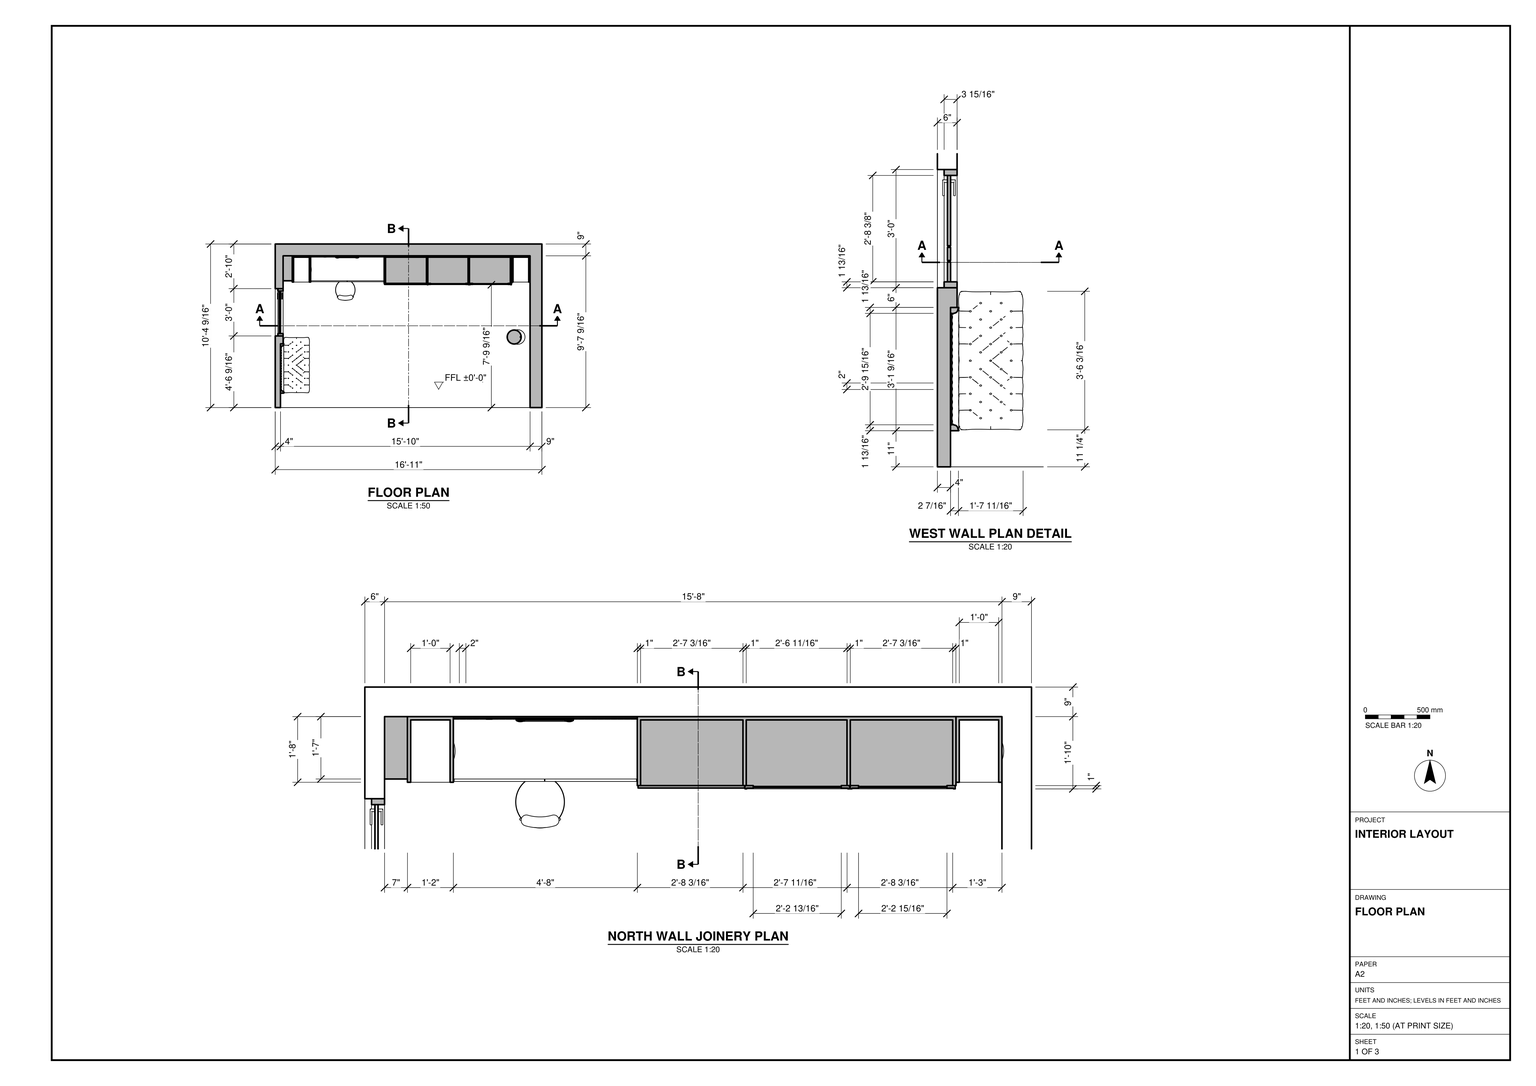
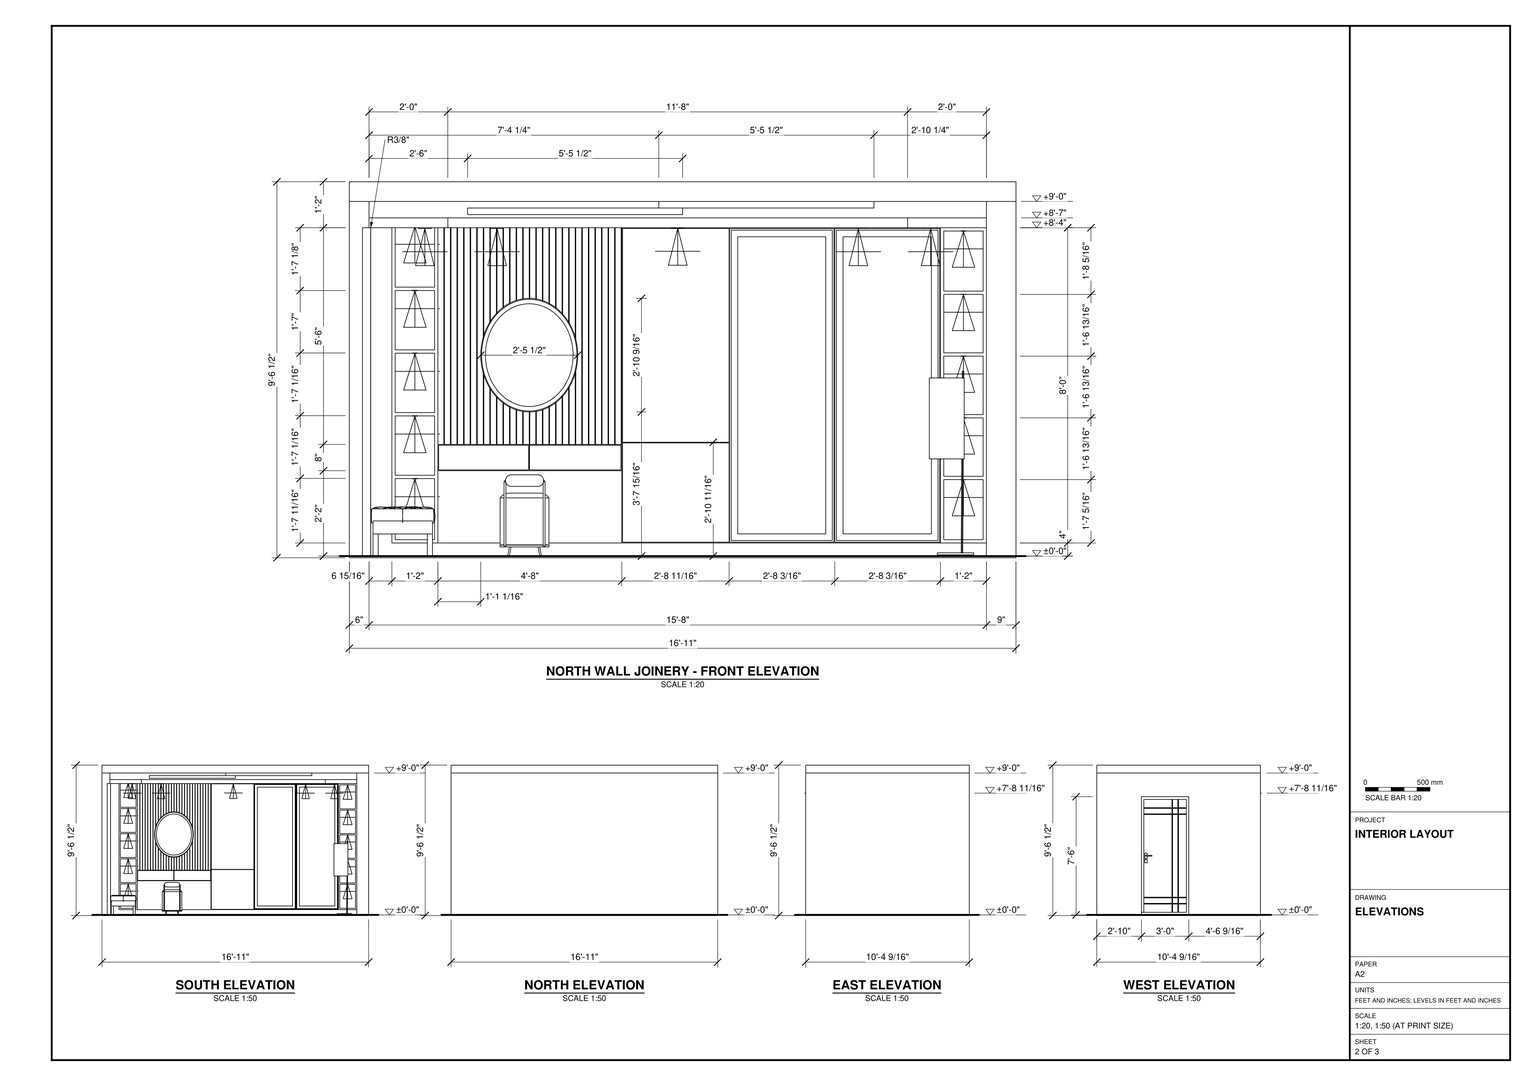
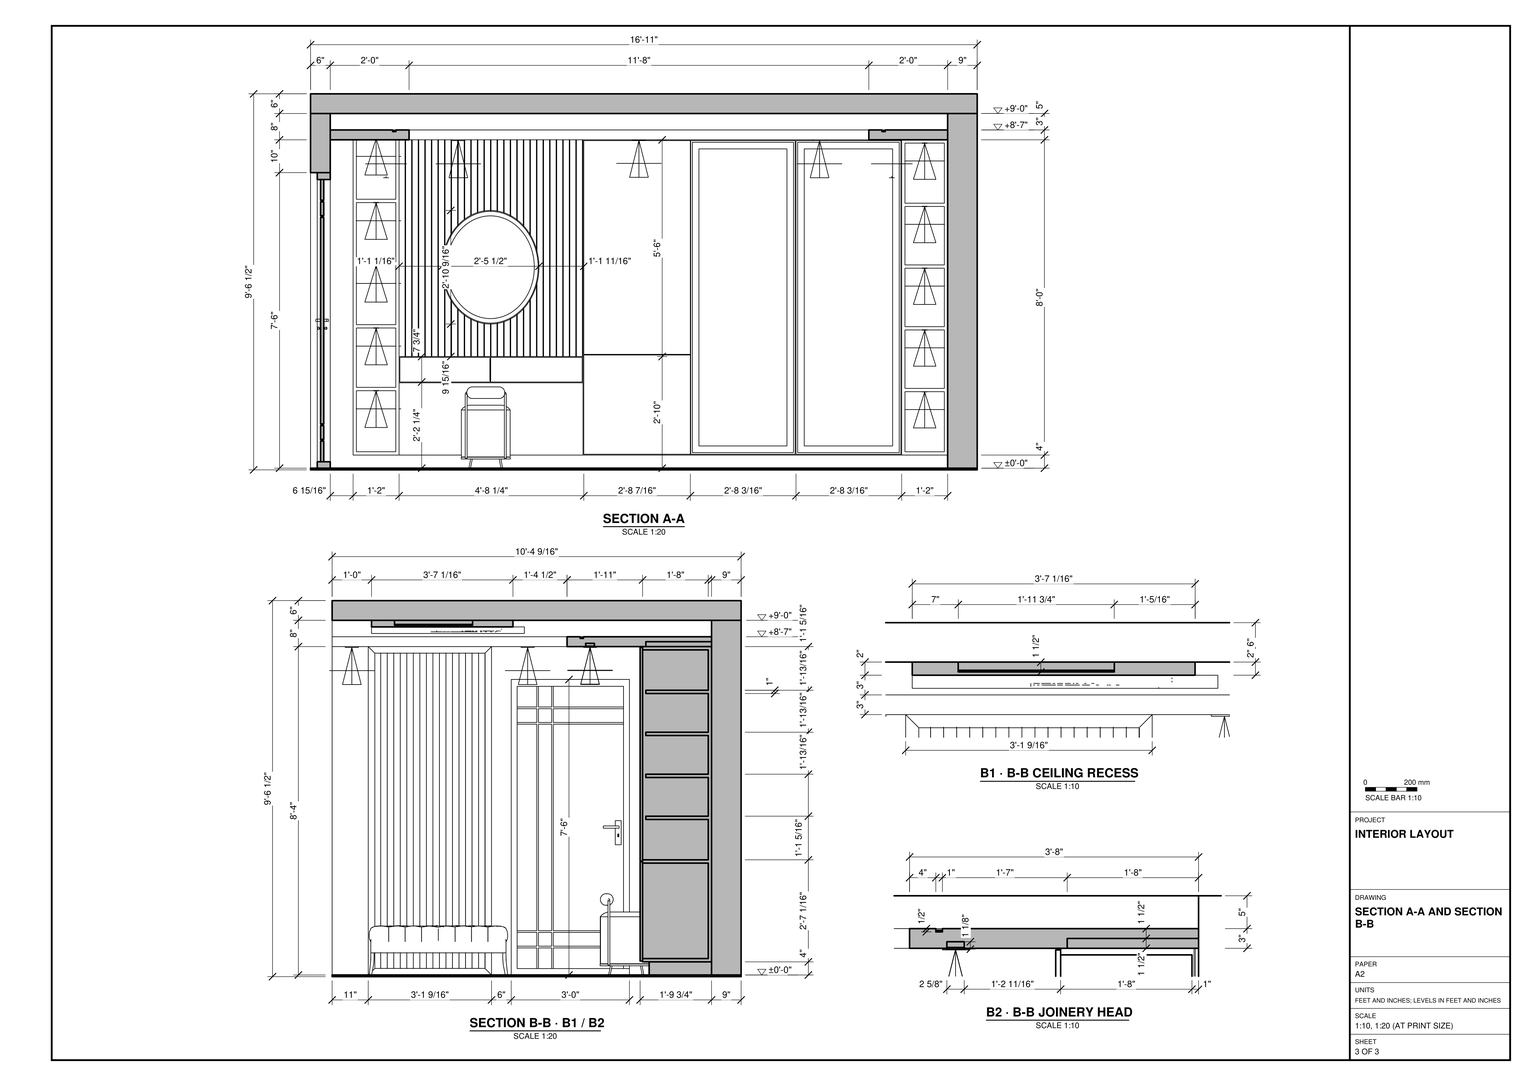
Work in feet and inches in SketchUp. Use task_files/diagram_01.pdf to model the dressing room. Set the finished floor at ±0'-0". The overall size is 16'-11" east to west, 10'-4 9/16" north to south and 9'-6 1/2" high.

Build the floor, the north, east and west walls, and the ceiling slab. Follow the wall thicknesses in plan and leave the south side open as drawn. Fit the door in the west wall, with the bench and its vertical slatted backing on the south side of the door.

Use the north wall joinery plan for cabinet depths and the front elevation for the arrangement of the bays. Model the dressing counter with drawers, knee space, a seat and a mirror on slatted backing. Continue the run with the tall cupboards and include the narrow open shelving at both ends. Use the sections to shape the plinth, joinery head and stepped ceiling recess. Place the lights as shown. Decor and loose items may be any suitable library components.

Keep shell elements and individual furniture and joinery pieces in separate groups or components, and use components for repeated parts. Save one SketchUp model as output_files/dressing_room_with_fitted_wardrobes_and_a_vanity.skp.

# SketchUp Ruby script. Lengths in inches.
U = 1.inch
M = Sketchup.active_model
def pt(a) = Geom::Point3d.new(a.map { |v| v * U })
def face(e, loops, mat)
  f = e.add_face(loops[0].map { |a| pt(a) })
  loops[1..].each { |l| e.add_face(l.map { |a| pt(a) }).erase! }
  f.material = f.back_material = mat if mat
  f
end
# faces: each face lists its corners as indices into pts; further lists are holes
def faces(e, pts, list, mat = nil) = list.each { |f| face(e, (f[0].is_a?(Array) ? f : [f]).map { |l| l.map { |i| pts[i] } }, mat) }
# xy, xz, yz: faces in a plane at the given z, y or x. An outline is a flat list of corners, or four numbers for a rectangle; further outlines are holes
def ring(l) = l.size == 4 ? [[l[0], l[1]], [l[2], l[1]], [l[2], l[3]], [l[0], l[3]]] : l.each_slice(2).to_a
def flat(e, list, mat, &to3) = list.each { |f| face(e, (f[0].is_a?(Array) ? f : [f]).map { |l| ring(l).map { |u, v| to3.(u, v) } }, mat) }
def xy(e, z, list, mat = nil) = flat(e, list, mat) { |x, y| [x, y, z] }
def xz(e, y, list, mat = nil) = flat(e, list, mat) { |x, z| [x, y, z] }
def yz(e, x, list, mat = nil) = flat(e, list, mat) { |y, z| [x, y, z] }
def lines(e, pts, list) = list.each { |a, b| e.add_line(pt(pts[a]), pt(pts[b])) }
# prism: a flat outline (further loops are holes) pulled along v
def prism(e, loops, v, mat = nil)
  f = face(e, loops, mat); d = Geom::Vector3d.new(v.map { |x| x * U })
  f.pushpull(f.normal.samedirection?(d) ? d.length : -d.length)
end
def box(e, o, s, mat = nil) = prism(e, [[o, [o[0] + s[0], o[1], o[2]], [o[0] + s[0], o[1] + s[1], o[2]], [o[0], o[1] + s[1], o[2]]]], [0, 0, s[2]], mat)
def at(x, y, z, deg = 0) = Geom::Transformation.translation(pt([x, y, z])) * Geom::Transformation.rotation(ORIGIN, Z_AXIS, deg.degrees)
def axes(o, x, y, z) = Geom::Transformation.new([*x, 0, *y, 0, *z, 0, *pt(o).to_a, 1])
def part(name) = M.definitions.add(name)
# library, detail: a bought-in or finely detailed component or shape, given as its bounding box
def library(name, o, s) = part(name).tap { |d| box(d.entities, o, s) }
def detail(e, o, s) = box(e.add_group.entities, o, s)
def put(e, d, t, mat = nil) = e.add_instance(d, t).tap { |i| i.material = mat if mat }
def group(e, t, mat = nil) = e.add_group.tap { |g| g.transformation = t; g.material = mat if mat }.entities
root = M.entities
M.materials.add("0001 AP 9436 AIR BREEZE").color = [243, 237, 232]
M.materials.add("[Color D01]").color = [255, 242, 204]
M.materials.add("[Color M08]").color = [30, 30, 30]
M.materials.add("[Marble Carrara Gold Floor Tile]").color = [236, 235, 232]
M.materials.add("[Metal Corrugated Shiny]1").color = [103, 84, 74]
M.materials.add("[Translucent Glass Gray]").color = [128, 128, 128]
M.materials["[Translucent Glass Gray]"].alpha = 0.5
M.materials.add("[Wood Cherry Original]").color = [109, 66, 38]
M.materials.add("[Wood Veneer 01]").color = [93, 54, 28]
c1 = library("Gwendolyn Accent Stool",[0,0,0],[15.91,14.93,24.75])
c2 = library("Component",[0,0,0],[66.93,19.69,17.91])
c3 = library("Untitled",[0,0,-1.87],[36,4.39,85.87])
c4 = part("modern minimalism stand lamp2")
prism(c4.entities,[[[6.34,1.24,0.43],[6.43,0.625,0.43],[6.46,0,0.43],[6.43,-0.625,0.43],[6.34,-1.24,0.43],[6.19,-1.85,0.43],[5.98,-2.4375,0.43],[5.72,-3,0.43],[5.4,-3.54,0.43],[5.04,-4.05,0.43],[4.625,-4.51,0.43],[4.17,-4.9375,0.43],[3.67,-5.32,0.43],[3.14,-5.65,0.43],[2.58,-5.92,0.43],[2,-6.15,0.43],[1.39,-6.31,0.43],[0.78,-6.41,0.43],[0.16,-6.46,0.43],[-0.47,-6.45,0.43],[-1.09,-6.37,0.43],[-1.7,-6.24,0.43],[-2.29,-6.04,0.43],[-2.86,-5.79,0.43],[-3.41,-5.49,0.43],[-3.92,-5.13,0.43],[-4.4,-4.73,0.43],[-4.84,-4.29,0.43],[-5.23,-3.8,0.43],[-5.57,-3.28,0.43],[-5.86,-2.72,0.43],[-6.1,-2.14,0.43],[-6.28,-1.55,0.43],[-6.4,-0.93,0.43],[-6.46,-0.3125,0.43],[-6.46,0.3125,0.43],[-6.4,0.93,0.43],[-6.28,1.55,0.43],[-6.1,2.14,0.43],[-5.86,2.72,0.43],[-5.57,3.28,0.43],[-5.23,3.8,0.43],[-4.84,4.29,0.43],[-4.4,4.73,0.43],[-3.92,5.13,0.43],[-3.41,5.49,0.43],[-2.86,5.79,0.43],[-2.29,6.04,0.43],[-1.7,6.24,0.43],[-1.09,6.37,0.43],[-0.47,6.45,0.43],[0.16,6.46,0.43],[0.78,6.41,0.43],[1.39,6.31,0.43],[2,6.15,0.43],[2.58,5.92,0.43],[3.14,5.65,0.43],[3.67,5.32,0.43],[4.17,4.9375,0.43],[4.625,4.51,0.43],[5.04,4.05,0.43],[5.4,3.54,0.43],[5.72,3,0.43],[5.98,2.4375,0.43],[6.19,1.85,0.43]]],[0,0,0.65],"[Color M08]")
p = [[4.66,0,0],[4.64,0.45,0],[4.58,0.9,0],[4.47,1.33,0],[4.32,1.76,0],[4.13,2.17,0],
  [3.9,2.56,0],[3.64,2.92,0],[3.34,3.26,0],[3.01,3.56,0],[2.65,3.84,0],[2.27,4.08,0],
  [1.86,4.28,0],[1.44,4.4375,0],[1.01,4.55,0],[0.5625,4.63,0],[0.11,4.66,0],[-0.34,4.65,0],
  [-0.79,4.6,0],[-1.23,4.5,0],[-1.65,4.36,0],[-2.07,4.18,0],[-2.46,3.96,0],[-2.83,3.71,0],
  [-3.18,3.42,0],[-3.49,3.09,0],[-3.77,2.74,0],[-4.02,2.36,0],[-4.23,1.97,0],[-4.4,1.55,0],
  [-4.53,1.12,0],[-4.62,0.67,0],[-4.66,0.23,0],[-4.66,-0.23,0],[-4.62,-0.67,0],[-4.53,-1.12,0],
  [-4.4,-1.55,0],[-4.23,-1.97,0],[-4.02,-2.36,0],[-3.77,-2.74,0],[-3.49,-3.09,0],[-3.18,-3.42,0],
  [-2.83,-3.71,0],[-2.46,-3.96,0],[-2.07,-4.18,0],[-1.65,-4.36,0],[-1.23,-4.5,0],[-0.79,-4.6,0],
  [-0.34,-4.65,0],[0.11,-4.66,0],[0.5625,-4.63,0],[1.01,-4.55,0],[1.44,-4.4375,0],[1.86,-4.28,0],
  [2.27,-4.08,0],[2.65,-3.84,0],[3.01,-3.56,0],[3.34,-3.26,0],[3.64,-2.92,0],[3.9,-2.56,0],
  [4.13,-2.17,0],[4.32,-1.76,0],[4.47,-1.33,0],[4.58,-0.9,0],[4.64,-0.45,0]]
lines(c4.entities,p,[[0,1],[1,2],[2,3],[3,4],[4,5],[5,6],[6,7],[7,8],[8,9],[9,10],[10,11],[11,12],
  [12,13],[13,14],[14,15],[15,16],[16,17],[17,18],[18,19],[19,20],[20,21],[21,22],[22,23],[23,24],
  [24,25],[25,26],[26,27],[27,28],[28,29],[29,30],[30,31],[31,32],[32,33],[33,34],[34,35],[35,36],
  [36,37],[37,38],[38,39],[39,40],[40,41],[41,42],[42,43],[43,44],[44,45],[45,46],[46,47],[47,48],
  [48,49],[50,51],[51,52],[52,53],[53,54],[54,55],[55,56],[56,57],[57,58],[58,59],[59,60],[60,61],
  [61,62],[62,63],[63,64],[64,0]])
g1 = group(c4.entities,at(2.28,0,0.76),"[Color M08]")
xy(g1,0,[[0,-0.28,-0.07,-0.27,-0.14,-0.24,-0.24,-0.14,-0.27,-0.07,-0.28,0,-0.27,0.07,-0.24,0.14,-0.14,0.24,-0.07,0.27,0,0.28,0.07,0.27,0.14,0.24,0.24,0.14,0.27,0.07,0.28,0,0.27,-0.07,0.24,-0.14,0.14,-0.24,0.07,-0.27]])
p = [[0.4,-0.28,59.29],[0.33,-0.27,59.29],[-0.07,-0.27,0],[0,-0.28,0],[0.26,-0.24,59.29],[-0.14,-0.24,0],
  [0.47,-0.27,59.29],[0.07,-0.27,0],[0.54,-0.24,59.29],[0.14,-0.24,0],[0.2,-0.19,59.29],[-0.19,-0.19,0],
  [0.16,-0.14,59.29],[-0.24,-0.14,0],[0.59,-0.19,59.29],[0.19,-0.19,0],[0.64,-0.14,59.28],[0.24,-0.14,0],
  [0.13,-0.07,59.29],[-0.27,-0.07,0],[0.12,0,59.29],[-0.28,0,0],[0.66,-0.07,59.28],[0.27,-0.07,0],
  [0.67,0,59.28],[0.28,0,0],[0.13,0.07,59.29],[-0.27,0.07,0],[0.66,0.07,59.28],[0.27,0.07,0],
  [0.16,0.14,59.29],[-0.24,0.14,0],[0.2,0.19,59.29],[-0.19,0.19,0],[0.59,0.19,59.29],[0.64,0.14,59.28],
  [0.24,0.14,0],[0.19,0.19,0],[0.26,0.24,59.29],[-0.14,0.24,0],[0.33,0.27,59.29],[-0.07,0.27,0],
  [0.47,0.27,59.29],[0.54,0.24,59.29],[0.14,0.24,0],[0.07,0.27,0],[0.4,0.28,59.29],[0,0.28,0],
  [0.4,0,59.29],[0,0,0]]
faces(g1,p,[[0,1,2,3],[1,4,5,2],[6,0,3,7],[8,6,7,9],[4,10,11,5],[10,12,13,11],[14,8,9,15],[16,14,15,17],
  [12,18,19,13],[18,20,21,19],[22,16,17,23],[24,22,23,25],[20,26,27,21],[28,24,25,29],[26,30,31,27],[30,32,33,31],
  [34,35,36,37],[35,28,29,36],[32,38,39,33],[38,40,41,39],[42,43,44,45],[43,34,37,44],[40,46,47,41],[46,42,45,47],
  [46,40,38,32,30,26,20,18,12,10,4,1,0,6,8,14,16,22,24,28,35,34,43,42]])
lines(g1,p,[[48,49]])
g2 = group(c4.entities,at(-9.28,-6.18,31.58))
yz(g2,0,[[5.88,0,6.48,26.3]],"[Color D01]")
p = [[5.13,0.09,0],[5.72,0.01,0],[5.72,0.01,26.3],[5.13,0.09,26.3],[6.32,0,0],[6.32,0,26.3],
  [6.92,0.04,0],[6.92,0.04,26.3],[7.51,0.14,0],[7.51,0.14,26.3],[4.55,0.22,0],[4.55,0.22,26.3],
  [8.08,0.3,0],[8.08,0.3,26.3],[3.98,0.4,0],[3.98,0.4,26.3],[8.64,0.51,0],[8.64,0.51,26.3],
  [3.43,0.64,0],[3.43,0.64,26.3],[9.17,0.78,0],[9.17,0.78,26.3],[2.91,0.93,0],[2.91,0.93,26.3],
  [9.68,1.09,0],[9.68,1.09,26.3],[2.42,1.27,0],[2.42,1.27,26.3],[10.16,1.45,0],[10.16,1.45,26.3],
  [1.96,1.65,0],[1.96,1.65,26.3],[10.59,1.86,0],[10.59,1.86,26.3],[1.55,2.08,0],[1.55,2.08,26.3],
  [10.99,2.31,0],[10.99,2.31,26.3],[1.17,2.55,0],[1.17,2.55,26.3],[11.34,2.79,0],[11.34,2.79,26.3],
  [0.85,3.04,0],[0.85,3.04,26.3],[11.64,3.31,0],[11.64,3.31,26.3],[0.57,3.57,0],[0.57,3.57,26.3],
  [11.89,3.85,0],[11.89,3.85,26.3],[0.34,4.125,0],[0.34,4.125,26.3],[12.09,4.41,0],[12.09,4.41,26.3],
  [0.17,4.7,0],[0.17,4.7,26.3],[12.24,4.99,0],[12.24,4.99,26.3],[0.06,5.28,0],[0.06,5.28,26.3],
  [12.32,5.58,0],[12.32,5.58,26.3],[0,5.88,0],[0,5.88,26.3],[12.35,6.18,0],[12.35,6.18,26.3],
  [12.32,6.77,0],[12.32,6.77,26.3],[0.06,7.07,0],[0,6.48,0],[0,6.48,26.3],[0.06,7.07,26.3],
  [12.24,7.36,0],[12.24,7.36,26.3],[0.17,7.66,0],[0.17,7.66,26.3],[12.09,7.94,0],[12.09,7.94,26.3],
  [0.34,8.23,0],[0.34,8.23,26.3],[11.89,8.51,0],[11.89,8.51,26.3],[0.57,8.78,0],[0.57,8.78,26.3],
  [11.64,9.05,0],[11.64,9.05,26.3],[0.85,9.31,0],[0.85,9.31,26.3],[11.34,9.5625,0],[11.34,9.5625,26.3],
  [1.17,9.81,0],[1.17,9.81,26.3],[10.99,10.05,0],[10.99,10.05,26.3],[1.55,10.27,0],[1.55,10.27,26.3],
  [10.59,10.49,0],[10.59,10.49,26.3],[1.96,10.7,0],[1.96,10.7,26.3],[10.16,10.9,0],[10.16,10.9,26.3],
  [2.42,11.09,0],[2.42,11.09,26.3],[9.68,11.26,0],[9.68,11.26,26.3],[2.91,11.43,0],[2.91,11.43,26.3],
  [9.17,11.58,0],[9.17,11.58,26.3],[3.43,11.72,0],[3.43,11.72,26.3],[8.64,11.84,0],[8.64,11.84,26.3],
  [3.98,11.95,0],[3.98,11.95,26.3],[8.08,12.05,0],[8.08,12.05,26.3],[4.55,12.14,0],[4.55,12.14,26.3],
  [5.13,12.27,0],[5.13,12.27,26.3],[7.51,12.21,0],[7.51,12.21,26.3],[6.92,12.3125,0],[6.92,12.3125,26.3],
  [5.72,12.34,0],[5.72,12.34,26.3],[6.32,12.35,0],[6.32,12.35,26.3]]
faces(g2,p,[[0,1,2,3],[1,4,5,2],[4,6,7,5],[6,8,9,7],[10,0,3,11],[8,12,13,9],[14,10,11,15],[12,16,17,13],
  [18,14,15,19],[16,20,21,17],[22,18,19,23],[20,24,25,21],[26,22,23,27],[24,28,29,25],[30,26,27,31],[28,32,33,29],
  [34,30,31,35],[32,36,37,33],[38,34,35,39],[36,40,41,37],[42,38,39,43],[40,44,45,41],[46,42,43,47],[44,48,49,45],
  [50,46,47,51],[48,52,53,49],[54,50,51,55],[52,56,57,53],[58,54,55,59],[56,60,61,57],[62,58,59,63],[60,64,65,61],
  [64,66,67,65],[68,69,70,71],[66,72,73,67],[74,68,71,75],[72,76,77,73],[78,74,75,79],[76,80,81,77],[82,78,79,83],
  [80,84,85,81],[86,82,83,87],[84,88,89,85],[90,86,87,91],[88,92,93,89],[94,90,91,95],[92,96,97,93],[98,94,95,99],
  [96,100,101,97],[102,98,99,103],[100,104,105,101],[106,102,103,107],[104,108,109,105],[110,106,107,111],[108,112,113,109],[114,110,111,115],
  [112,116,117,113],[118,114,115,119],[120,118,119,121],[116,122,123,117],[122,124,125,123],[126,120,121,127],[128,126,127,129],[124,128,129,125]],"[Color D01]")
c5 = library("5",[-0.54,0,0],[15.08,96,20])
c6 = library("Group\#5",[0,0,0],[56,97.5,19.75])
c7 = library("2",[0,0,0],[30.68,94,19])
c8 = part("3")
xy(c8.entities,0,[[[0,0,31.43,94.75],[2.47,2.5,28.96,92.25]]])
xy(c8.entities,0.75,[[[0.49,0.5,30.9375,94.25],[2.47,2.5,28.96,92.25]]])
xy(c8.entities,1,[[[0,0,31.43,94.75],[0.49,0.5,30.9375,94.25]]])
xz(c8.entities,0,[[0,0,31.43,1]])
xz(c8.entities,0.5,[[0.49,0.75,30.9375,1]])
xz(c8.entities,2.5,[[2.47,0,28.96,0.75]])
xz(c8.entities,92.25,[[2.47,0,28.96,0.75]])
xz(c8.entities,94.25,[[0.49,0.75,30.9375,1]])
xz(c8.entities,94.75,[[0,0,31.43,1]])
yz(c8.entities,0,[[0,0,94.75,1]])
yz(c8.entities,0.49,[[0.5,0.75,94.25,1]])
yz(c8.entities,2.47,[[2.5,0,92.25,0.75]])
yz(c8.entities,28.96,[[2.5,0,92.25,0.75]])
yz(c8.entities,30.9375,[[0.5,0.75,94.25,1]])
yz(c8.entities,31.43,[[0,0,94.75,1]])
g3 = group(c8.entities,at(2.47,2.5,0.28))
box(g3,[0,0,0],[26.49,89.75,0.2],"[Translucent Glass Gray]")
c9 = library("Group\#15",[59.8,0,0],[2.53,37.54,100])
c10 = library("Group\#18",[0,-96.36,-11.56],[188,116.36,14.56])
c11 = library("Group\#21",[0,0,-6],[123.75,46.54,4])
put(root,c1,at(45.89,97.51,1.5,-90))
g4 = group(root,at(0,11,1))
put(g4,c2,axes([6.42,42.45,0.5],[0,-0.63,0],[1,0,0],[0,0,0.84]))
g5 = group(g4,at(-3,0,0.5))
xy(g5,0,[[197,-11,197,104.54,9,104.54,9,79.54,3,79.54,3,113.54,206,113.54,206,-11],[3,-11,3,43.54,9,43.54,9,37.54,7,37.54,7,-11]])
xy(g5,90,[[3,43.54,9,79.54]])
xy(g5,100,[[7,-11,9,37.54]])
xy(g5,108,[[3,-11,9,-11,9,104.54,197,104.54,197,-11,206,-11,206,113.54,3,113.54]])
xz(g5,-11,[[3,0,7,0,7,100,9,100,9,108,3,108],[197,0,206,108]])
xz(g5,37.54,[[7,0,9,100]])
xz(g5,43.54,[[3,0,9,90]])
xz(g5,79.54,[[3,0,9,90]])
xz(g5,104.54,[[9,0,197,108]])
xz(g5,113.54,[[3,0,206,108]])
yz(g5,3,[[-11,0,-11,108,113.54,108,113.54,0,79.54,0,79.54,90,43.54,90,43.54,0]])
yz(g5,7,[[-11,0,37.54,100]])
yz(g5,9,[[37.54,0,43.54,0,43.54,90,79.54,90,79.54,0,104.54,0,104.54,108,-11,108,-11,100,37.54,100]],"0001 AP 9436 AIR BREEZE")
yz(g5,197,[[-11,0,104.54,108]],"0001 AP 9436 AIR BREEZE")
yz(g5,206,[[-11,0,113.54,108]])
put(g5,c3,axes([4.61,79.54,1.96],[0,-1,0],[1,0,0],[0,0,1.04814]))
put(g5,c4,axes([187.59,42.73,0],[0.86,0,0],[0,0.86,0],[0,0,0.9374]))
g6 = group(g5,at(9,104.54,0))
xz(g6,0,[[0,0,188,108]])
put(g6,c5,axes([6.96,0,4],[1,0,0],[0,0,1.01562],[0,-1,0]),"0001 AP 9436 AIR BREEZE")
put(g6,c5,axes([174,0,4],[1,0,0],[0,0,1],[0,-1,0]),"0001 AP 9436 AIR BREEZE")
put(g6,c6,axes([20.96,0,4],[1,0,0],[0,0,1],[0,-1,0]))
g7 = group(g6,at(76.96,0,4))
xy(g7,0,[[0,-21,97.04,0]],"[Wood Veneer 01]")
xy(g7,1,[[33.18,-21,63.86,-1],[64.86,-21,96.04,-1]],"0001 AP 9436 AIR BREEZE")
xy(g7,1,[[1,-21,32.18,-1]],"[Wood Veneer 01]")
xy(g7,30.07,[[1,-21,32.18,-1]],"[Wood Veneer 01]")
xy(g7,31.07,[[1,-21,32.18,-1]],"[Wood Veneer 01]")
xy(g7,43.35,[[1,-20,32.18,-1]],"[Wood Veneer 01]")
xy(g7,44.35,[[1,-20,32.18,-1]],"[Wood Veneer 01]")
xy(g7,56.14,[[1,-20,32.18,-1]],"[Wood Veneer 01]")
xy(g7,57.14,[[1,-20,32.18,-1]],"[Wood Veneer 01]")
xy(g7,68.93,[[1,-20,32.18,-1]],"[Wood Veneer 01]")
xy(g7,69.93,[[1,-20,32.18,-1]],"[Wood Veneer 01]")
xy(g7,81.71,[[1,-20,32.18,-1]],"[Wood Veneer 01]")
xy(g7,82.71,[[1,-20,32.18,-1]],"[Wood Veneer 01]")
xy(g7,95,[[33.18,-21,63.86,-1],[64.86,-21,96.04,-1]],"0001 AP 9436 AIR BREEZE")
xy(g7,95,[[1,-21,32.18,-1]],"[Wood Veneer 01]")
xy(g7,96,[[0,-21,97.04,0]],"[Wood Veneer 01]")
xz(g7,-21,[[[0,0,97.04,96],[64.86,1,96.04,95],[33.18,1,63.86,95],[1,31.07,32.18,95],[1,1,32.18,30.07]]],"[Wood Veneer 01]")
xz(g7,-20,[[1,43.35,32.18,44.35],[1,56.14,32.18,57.14],[1,68.93,32.18,69.93],[1,81.71,32.18,82.71]],"[Wood Veneer 01]")
xz(g7,-1,[[64.86,1,96.04,95]],"0001 AP 9436 AIR BREEZE")
xz(g7,-1,[[1,1,32.18,30.07],[1,31.07,32.18,43.35],[1,44.35,32.18,56.14],[1,57.14,32.18,68.93],[1,69.93,32.18,81.71],
  [1,82.71,32.18,95]],"[Wood Veneer 01]")
xz(g7,0,[[0,0,97.04,96]],"[Wood Veneer 01]")
yz(g7,0,[[-21,0,0,96]],"[Wood Veneer 01]")
yz(g7,1,[[-21,1,-1,30.07],[-21,31.07,-1,31.07,-1,43.35,-20,43.35,-20,44.35,-1,44.35,-1,56.14,-20,56.14,-20,57.14,-1,57.14,-1,68.93,-20,68.93,-20,69.93,-1,69.93,-1,81.71,-20,81.71,-20,82.71,-1,82.71,-1,95,-21,95]],"[Wood Veneer 01]")
yz(g7,32.18,[[-21,1,-1,30.07],[-21,31.07,-21,95,-1,95,-1,82.71,-20,82.71,-20,81.71,-1,81.71,-1,69.93,-20,69.93,-20,68.93,-1,68.93,-1,57.14,-20,57.14,-20,56.14,-1,56.14,-1,44.35,-20,44.35,-20,43.35,-1,43.35,-1,31.07]],"[Wood Veneer 01]")
yz(g7,33.18,[[-21,1,-1,95]],"0001 AP 9436 AIR BREEZE")
yz(g7,63.86,[[-21,1,-1,95]],"0001 AP 9436 AIR BREEZE")
yz(g7,64.86,[[-21,1,-1,95]],"0001 AP 9436 AIR BREEZE")
yz(g7,96.04,[[-21,1,-1,95]],"0001 AP 9436 AIR BREEZE")
yz(g7,97.04,[[-21,0,0,96]],"[Wood Veneer 01]")
put(g7,c7,axes([33.18,-1,1],[1,0,0],[0,0,1],[0,-1,0]),"0001 AP 9436 AIR BREEZE")
put(g7,c7,axes([64.86,-1,1],[1.0163,0,0],[0,0,1],[0,-1,0]),"0001 AP 9436 AIR BREEZE")
put(g7,c8,axes([32.8,-21,0.25],[1.01193,0,0],[0,0,1.00792],[0,-1,0]),"[Metal Corrugated Shiny]1")
put(g7,c8,axes([64.86,-21,0.25],[1.0163,0,0],[0,0,1.00792],[0,-1,0]),"[Metal Corrugated Shiny]1")
g8 = group(g7,at(1,-21,1),"[Wood Cherry Original]")
xy(g8,-0.75,[[-0.75,-0.75,31.68,0]])
xy(g8,29.47,[[-0.75,-0.75,31.68,0]])
xy(g8,29.67,[[-0.75,-0.75,31.68,0]])
xy(g8,94.75,[[-0.75,-0.75,31.68,0]])
xz(g8,-0.75,[[-0.75,-0.75,31.68,29.47],[-0.75,29.67,31.68,94.75]],"[Wood Cherry Original]")
xz(g8,0,[[-0.75,-0.75,31.68,29.47],[-0.75,29.67,31.68,94.75]])
yz(g8,-0.75,[[-0.75,-0.75,0,29.47],[-0.75,29.67,0,94.75]])
yz(g8,31.68,[[-0.75,-0.75,0,29.47],[-0.75,29.67,0,94.75]])
g9 = group(g5,at(15.96,104.54,0),"0001 AP 9436 AIR BREEZE")
prism(g9,[[[181.04,0,4],[181.04,0,0],[-6.96,0,0],[-6.96,0,100],[0,0,100],[0,0,4]]],[0,-19,0])
put(g5,c9,at(-52.8,0,0),"0001 AP 9436 AIR BREEZE")
put(g5,c10,at(9,84.54,100))
g10 = group(g5,at(9,104.54,108))
box(g10,[-6,-115.54,0],[203,124.54,6])
put(g10,c11,at(30,-103.54,2))
g11 = group(g5,at(3,-11,-0.5))
xy(g11,0,[[0,0,203,124.54]])
xy(g11,0.5,[[0,0,203,124.54]],"[Marble Carrara Gold Floor Tile]")
xz(g11,0,[[0,0,203,0.5]])
xz(g11,124.54,[[0,0,203,0.5]])
yz(g11,0,[[0,0,124.54,0.5]])
yz(g11,203,[[0,0,124.54,0.5]])
